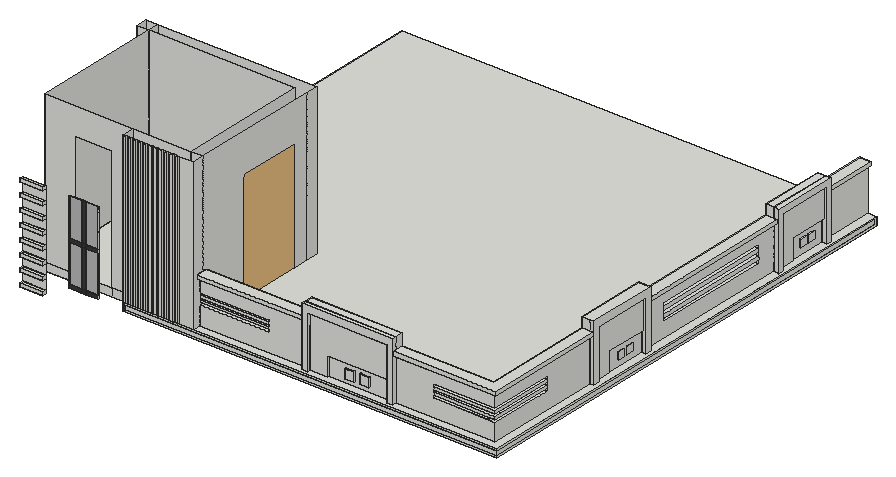
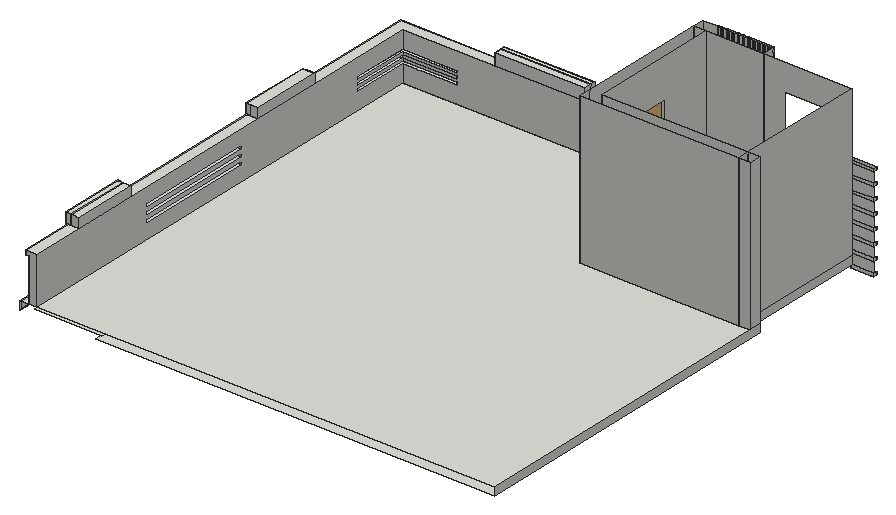
# SketchUp Ruby script. Lengths in inches.
U = 1.inch
M = Sketchup.active_model
def pt(a) = Geom::Point3d.new(a.map { |v| v * U })
def face(e, loops, mat)
  f = e.add_face(loops[0].map { |a| pt(a) })
  loops[1..].each { |l| e.add_face(l.map { |a| pt(a) }).erase! }
  f.material = f.back_material = mat if mat
  f
end
# faces: each face lists its corners as indices into pts; further lists are holes
def faces(e, pts, list, mat = nil) = list.each { |f| face(e, (f[0].is_a?(Array) ? f : [f]).map { |l| l.map { |i| pts[i] } }, mat) }
# xy, xz, yz: faces in a plane at the given z, y or x. An outline is a flat list of corners, or four numbers for a rectangle; further outlines are holes
def ring(l) = l.size == 4 ? [[l[0], l[1]], [l[2], l[1]], [l[2], l[3]], [l[0], l[3]]] : l.each_slice(2).to_a
def flat(e, list, mat, &to3) = list.each { |f| face(e, (f[0].is_a?(Array) ? f : [f]).map { |l| ring(l).map { |u, v| to3.(u, v) } }, mat) }
def xy(e, z, list, mat = nil) = flat(e, list, mat) { |x, y| [x, y, z] }
def xz(e, y, list, mat = nil) = flat(e, list, mat) { |x, z| [x, y, z] }
def yz(e, x, list, mat = nil) = flat(e, list, mat) { |y, z| [x, y, z] }
def lines(e, pts, list) = list.each { |a, b| e.add_line(pt(pts[a]), pt(pts[b])) }
# prism: a flat outline (further loops are holes) pulled along v
def prism(e, loops, v, mat = nil)
  f = face(e, loops, mat); d = Geom::Vector3d.new(v.map { |x| x * U })
  f.pushpull(f.normal.samedirection?(d) ? d.length : -d.length)
end
def box(e, o, s, mat = nil) = prism(e, [[o, [o[0] + s[0], o[1], o[2]], [o[0] + s[0], o[1] + s[1], o[2]], [o[0], o[1] + s[1], o[2]]]], [0, 0, s[2]], mat)
def at(x, y, z, deg = 0) = Geom::Transformation.translation(pt([x, y, z])) * Geom::Transformation.rotation(ORIGIN, Z_AXIS, deg.degrees)
def axes(o, x, y, z) = Geom::Transformation.new([*x, 0, *y, 0, *z, 0, *pt(o).to_a, 1])
def part(name) = M.definitions.add(name)
# library, detail: a bought-in or finely detailed component or shape, given as its bounding box
def library(name, o, s) = part(name).tap { |d| box(d.entities, o, s) }
def detail(e, o, s) = box(e.add_group.entities, o, s)
def put(e, d, t, mat = nil) = e.add_instance(d, t).tap { |i| i.material = mat if mat }
def group(e, t, mat = nil) = e.add_group.tap { |g| g.transformation = t; g.material = mat if mat }.entities
root = M.entities
M.materials.add("[Color M07]").color = [58, 58, 58]
M.materials.add("[Mirror 01]").color = [185, 185, 185]
c1 = library("Door 243 053",[-21.6,-2.79,-0.07],[43.2,5.58,82.64])
xy(root,237.07,[[7.9375,22.5,25.22,25.1875]])
xy(root,239.42,[[7.9375,22.5,25.22,25.1875]])
xy(root,244.8125,[[357.6875,206.85,364.9375,220.375],[364.9375,206.85,367,220.375]])
xy(root,246,[[84.23,24.75,84.23,25.1875,367.9375,25.1875,367.9375,385.1875,368.375,385.1875,368.375,24.75],[84.23,25.1875,137.39,34.1875],[196.07,25.625,215.37,31.1875],[327.58,25.625,343.4,25.625,343.4,28.1875,359.0625,28.1875,359.0625,31.1875,327.58,31.1875],[359.0625,28.1875,361.9375,31.1875],
  [361.9375,28.1875,364.9375,31.1875],[137.39,31.1875,137.39,34.1875,84.23,34.1875,84.23,133.1875,310.9375,133.1875,310.9375,379.1875,361.9375,379.1875,361.9375,34.1875,343.4,34.1875,343.4,36.25,327.58,36.25,327.58,31.1875,215.37,31.1875,215.37,36.25,196.07,36.25,196.07,31.1875],[196.07,31.1875,215.37,36.25],[327.58,31.1875,361.9375,31.1875,361.9375,34.1875,343.4,34.1875,343.4,36.25,327.58,36.25],[16.9375,34.1875,84.23,133.1875],
  [[7.9375,133.1875,310.9375,385.1875],[16.9375,142.1875,301.9375,376.1875]]])
xy(root,247,[[85.23,24.75,368.375,24.75,368.375,384.1875,367.9375,384.1875,367.9375,25.1875,85.23,25.1875],[364.9375,70.91,367,84.5]])
xy(root,247.11,[[52.28,25.1875,55.28,26.1875],[43.02,25.6875,52.28,26.1875],[55.28,25.6875,64.8,26.1875]])
xy(root,247.11,[[43.02,25.1875,52.28,25.6875],[55.28,25.1875,64.8,25.6875]],"[Color M07]")
xy(root,247.25,[[7.9375,22.5,25.22,25.1875]])
xy(root,249.6,[[7.9375,22.5,25.22,25.1875]])
xy(root,249.74,[[52.28,25.1875,55.28,26.1875],[43.02,25.6875,52.28,26.1875],[55.28,25.6875,64.8,26.1875]])
xy(root,249.74,[[43.02,25.1875,52.28,25.6875],[55.28,25.1875,64.8,25.6875]],"[Color M07]")
xy(root,251,[[84.23,24.75,85.23,25.1875],[85.23,24.75,85.23,25.1875,367.9375,25.1875,367.9375,384.1875,368.375,384.1875,368.375,24.75]])
xy(root,252,[[84.23,24.75,85.23,25.1875],[85.23,24.75,368.375,24.75,368.375,385.1875,367.9375,385.1875,367.9375,25.1875,85.23,25.1875],[84.23,25.1875,128.39,34.1875],[128.39,25.1875,137.39,34.1875],[137.39,25.1875,367.9375,25.1875,367.9375,385.1875,361.9375,385.1875,361.9375,344.85,366.25,344.85,366.25,341.21,361.9375,341.21,361.9375,312.14,363.5,312.14,363.5,299.05,366.25,299.05,366.25,295.41,361.9375,295.41,361.9375,174.68,365.1875,174.68,365.1875,170.17,361.9375,170.17,361.9375,137.91,363.125,137.91,363.125,125.76,365.1875,125.76,365.1875,121.25,361.9375,121.25,361.9375,31.1875,286.38,31.1875,286.38,27.9375,282.22,27.9375,282.22,31.1875,235.34,31.1875,235.34,30.125,221.92,30.125,221.92,27.9375,217.77,27.9375,217.77,31.1875,137.39,31.1875],
  [217.77,27.9375,221.92,31.1875],[282.22,27.9375,286.38,31.1875],[221.92,30.125,221.92,31.1875,137.39,31.1875,137.39,37.1875,361.9375,37.1875,361.9375,31.1875,235.34,31.1875,235.34,30.125],[16.9375,34.1875,84.23,133.1875],[84.23,34.1875,128.39,133.1875],
  [128.39,34.1875,137.39,73.1875],[137.39,37.1875,355.9375,37.1875,355.9375,385.1875,7.9375,385.1875,7.9375,142.1875,137.39,142.1875,137.39,121.1875,128.39,121.1875,128.39,73.1875,137.39,73.1875],[355.9375,37.1875,355.9375,385.1875,361.9375,385.1875,361.9375,312.14,363.5,312.14,363.5,299.05,361.9375,299.05,361.9375,137.91,363.125,137.91,363.125,125.76,361.9375,125.76,361.9375,37.1875],[128.39,121.1875,137.39,133.1875],[361.9375,121.25,365.1875,125.76],
  [7.9375,133.1875,16.9375,142.1875],[16.9375,133.1875,137.39,142.1875],[361.9375,170.17,365.1875,174.68],[361.9375,295.41,366.25,299.05],[361.9375,341.21,366.25,344.85]])
xy(root,252.6875,[[84.23,24.25,86.79,25.1875],[88.1,24.25,90.66,25.1875],[91.98,24.25,94.54,25.1875],[95.85,24.25,98.41,25.1875],[99.73,24.25,102.29,25.1875],
  [103.6,24.25,106.16,25.1875],[107.48,24.25,110.04,25.1875],[111.35,24.25,113.91,25.1875],[115.54,24.25,118.1,25.1875],[119.73,24.25,122.29,25.1875],
  [123.91,24.25,126.48,25.1875]])
xy(root,255.53,[[248.55,30.125,255.49,31.1875],[259.49,30.125,266.43,31.1875]])
xy(root,257.23,[[361.9375,146.76,363.125,152.14],[361.9375,154.89,363.125,160.26]])
xy(root,257.44,[[7.9375,22.5,25.22,25.1875]])
xy(root,257.85,[[361.9375,319.64,363.5,325.27],[361.9375,327.39,363.5,333.02]])
xy(root,259.79,[[7.9375,22.5,25.22,25.1875]])
xy(root,262.46,[[248.55,30.125,255.49,31.1875],[259.49,30.125,266.43,31.1875]])
xy(root,262.6,[[361.9375,146.76,363.125,152.14],[361.9375,154.89,363.125,160.26]])
xy(root,263.41,[[355.9375,190.16,361.9375,281.48]])
xy(root,263.48,[[361.9375,319.64,363.5,325.27],[361.9375,327.39,363.5,333.02]])
xy(root,265.05,[[314.9375,31.1875,355.9375,37.1875],[355.9375,31.1875,361.9375,80.6875]])
xy(root,266.06,[[355.9375,190.16,361.9375,281.48]])
xy(root,266.25,[[235.34,30.125,282.22,31.1875]])
xy(root,266.44,[[137.39,31.1875,189.76,34.1875]])
xy(root,267.01,[[314.9375,31.1875,355.9375,37.1875],[355.9375,31.1875,361.9375,80.6875]])
xy(root,267.0625,[[361.9375,137.91,363.125,170.17]])
xy(root,267.63,[[7.9375,22.5,25.22,25.1875]])
xy(root,267.875,[[361.9375,312.14,363.5,341.21]])
xy(root,268.03,[[137.39,31.1875,189.76,34.1875]])
xy(root,268.71,[[355.9375,190.16,361.9375,281.48]])
xy(root,268.97,[[314.9375,31.1875,361.9375,37.1875],[355.9375,37.1875,361.9375,80.6875]])
xy(root,269.62,[[137.39,31.1875,189.76,34.1875]])
xy(root,269.98,[[7.9375,22.5,25.22,25.1875]])
xy(root,270.94,[[314.9375,31.1875,361.9375,37.1875],[355.9375,37.1875,361.9375,80.6875]])
xy(root,271.2,[[137.39,31.1875,189.76,34.1875]])
xy(root,271.36,[[355.9375,190.16,361.9375,281.48]])
xy(root,272.79,[[137.39,31.1875,189.76,34.1875]])
xy(root,272.9,[[314.9375,31.1875,355.9375,37.1875],[355.9375,31.1875,361.9375,80.6875]])
xy(root,274.01,[[355.9375,190.16,361.9375,281.48]])
xy(root,274.38,[[137.39,31.1875,189.76,34.1875]])
xy(root,274.86,[[314.9375,31.1875,355.9375,37.1875],[355.9375,31.1875,361.9375,80.6875]])
xy(root,276.66,[[355.9375,190.16,361.9375,281.48]])
xy(root,277.82,[[7.9375,22.5,25.22,25.1875]])
xy(root,278.42,[[52.28,25.1875,55.28,26.1875],[43.02,25.6875,52.28,26.1875],[55.28,25.6875,64.8,26.1875]])
xy(root,278.42,[[43.02,25.1875,52.28,25.6875],[55.28,25.1875,64.8,25.6875]],"[Color M07]")
xy(root,280.17,[[7.9375,22.5,25.22,25.1875]])
xy(root,281.05,[[52.28,25.1875,55.28,26.1875],[43.02,25.5,52.28,25.6875],[55.28,25.5,64.8,25.6875],[43.02,25.6875,52.28,26.1875],[55.28,25.6875,64.8,26.1875]])
xy(root,281.05,[[43.02,25.1875,52.28,25.5],[55.28,25.1875,64.8,25.5]],"[Color M07]")
xy(root,285,[[137.39,28.6875,217.77,31.1875],[286.38,28.6875,364.4375,31.1875],[361.9375,31.1875,364.4375,121.25],[361.9375,174.68,364.4375,295.41],[361.9375,344.85,364.4375,385.1875]])
xy(root,288,[[7.9375,22.5,25.22,25.1875],[137.39,28.6875,217.77,37.1875],[286.38,28.6875,364.4375,28.6875,364.4375,121.25,355.9375,121.25,355.9375,37.1875,286.38,37.1875],[217.77,31.1875,286.38,37.1875],[355.9375,121.25,361.9375,174.68],
  [355.9375,174.68,364.4375,295.41],[355.9375,344.85,364.4375,385.1875]])
xy(root,289.87,[[363.125,125.76,365.1875,170.17]])
xy(root,290.35,[[7.9375,22.5,25.22,25.1875]])
xy(root,290.6875,[[361.9375,299.05,363.5,341.21],[363.5,299.05,366.25,341.21]])
xy(root,291.53,[[221.92,27.9375,282.22,30.125]])
xy(root,295.4375,[[355.9375,121.25,365.1875,174.68],[355.9375,295.41,361.9375,344.85],[361.9375,295.41,366.25,344.85]])
xy(root,296.9375,[[217.77,27.9375,286.38,31.1875],[217.77,31.1875,286.38,37.1875]])
xy(root,298.19,[[7.9375,22.5,25.22,25.1875]])
xy(root,300.54,[[7.9375,22.5,25.22,25.1875]])
xy(root,308.38,[[7.9375,22.5,25.22,25.1875]])
xz(root,22.5,[[7.9375,237.07,25.22,239.42],[7.9375,247.25,25.22,249.6],[7.9375,257.44,25.22,259.79],[7.9375,267.63,25.22,269.98],[7.9375,277.82,25.22,280.17],
  [7.9375,288,25.22,290.35],[7.9375,298.19,25.22,300.54],[7.9375,308.38,25.22,310.73]])
xz(root,24.25,[[84.23,252.6875,86.79,366],[88.1,252.6875,90.66,366],[91.98,252.6875,94.54,366],[95.85,252.6875,98.41,366],[99.73,252.6875,102.29,366],
  [103.6,252.6875,106.16,366],[107.48,252.6875,110.04,366],[111.35,252.6875,113.91,366],[115.54,252.6875,118.1,366],[119.73,252.6875,122.29,366],
  [123.91,252.6875,126.48,366]])
xz(root,24.75,[[84.23,246,368.375,246,368.375,247,85.23,247,85.23,251,84.23,251],[84.23,251,85.23,252],[85.23,251,368.375,252]])
xz(root,25.1875,[[7.9375,237.07,25.22,239.42],[7.9375,239.42,25.22,247.25],[85.23,247,367.9375,251],[7.9375,247.25,25.22,249.6],[7.9375,249.6,25.22,257.44],
  [84.23,251,85.23,252],[84.23,252,137.39,252,137.39,366,126.48,366,126.48,252.6875,123.91,252.6875,123.91,366,122.29,366,122.29,252.6875,119.73,252.6875,119.73,366,118.1,366,118.1,252.6875,115.54,252.6875,115.54,366,113.91,366,113.91,252.6875,111.35,252.6875,111.35,366,110.04,366,110.04,252.6875,107.48,252.6875,107.48,366,106.16,366,106.16,252.6875,103.6,252.6875,103.6,366,102.29,366,102.29,252.6875,99.73,252.6875,99.73,366,98.41,366,98.41,252.6875,95.85,252.6875,95.85,366,94.54,366,94.54,252.6875,91.98,252.6875,91.98,366,90.66,366,90.66,252.6875,88.1,252.6875,88.1,366,86.79,366,86.79,252.6875,84.23,252.6875],[84.23,252.6875,86.79,366],[88.1,252.6875,90.66,366],[91.98,252.6875,94.54,366],
  [95.85,252.6875,98.41,366],[99.73,252.6875,102.29,366],[103.6,252.6875,106.16,366],[107.48,252.6875,110.04,366],[111.35,252.6875,113.91,366],
  [115.54,252.6875,118.1,366],[119.73,252.6875,122.29,366],[123.91,252.6875,126.48,366],[7.9375,257.44,25.22,259.79],[7.9375,259.79,25.22,267.63],
  [7.9375,267.63,25.22,269.98],[7.9375,269.98,25.22,277.82],[7.9375,277.82,25.22,280.17],[7.9375,280.17,25.22,288],[7.9375,288,25.22,290.35],
  [7.9375,290.35,25.22,298.19],[7.9375,298.19,25.22,300.54],[7.9375,300.54,25.22,308.38],[7.9375,308.38,25.22,310.73]])
xz(root,25.1875,[[43.02,247.11,52.28,249.74],[52.28,247.11,55.28,249.74],[55.28,247.11,64.8,249.74],[52.28,249.74,55.28,278.42],[43.02,278.42,52.28,281.05],
  [52.28,278.42,55.28,281.05],[55.28,278.42,64.8,281.05],[52.28,281.05,55.28,309.73]],"[Color M07]")
xz(root,25.5,[[43.02,281.05,52.28,309.73],[55.28,281.05,64.8,309.73]],"[Mirror 01]")
xz(root,25.6875,[[43.02,281.05,52.28,309.73],[55.28,281.05,64.8,309.73]])
xz(root,25.6875,[[43.02,249.74,52.28,278.42],[55.28,249.74,64.8,278.42]],"[Mirror 01]")
xz(root,26.1875,[[43.02,247.11,52.28,249.74],[52.28,247.11,55.28,249.74],[55.28,247.11,64.8,249.74],[52.28,249.74,55.28,278.42],[43.02,278.42,52.28,281.05],
  [52.28,278.42,55.28,281.05],[55.28,278.42,64.8,281.05],[52.28,281.05,55.28,309.73]],"[Color M07]")
xz(root,26.1875,[[43.02,249.74,52.28,278.42],[55.28,249.74,64.8,278.42],[43.02,281.05,52.28,309.73],[55.28,281.05,64.8,309.73]],"[Mirror 01]")
xz(root,27.9375,[[217.77,252,221.92,252,221.92,291.53,282.22,291.53,282.22,252,286.38,252,286.38,296.9375,217.77,296.9375]])
xz(root,28.6875,[[137.39,285,217.77,288],[286.38,285,364.4375,288]])
xz(root,30.125,[[221.92,252,235.34,252,235.34,266.25,282.22,266.25,282.22,291.53,221.92,291.53],[248.55,255.53,255.49,262.46],[259.49,255.53,266.43,262.46]])
xz(root,31.1875,[[137.39,252,217.77,252,217.77,285,137.39,285,137.39,274.38,189.76,274.38,189.76,266.44,137.39,266.44],[217.77,252,217.77,288,286.38,288,286.38,252,282.22,252,282.22,283.84,221.92,283.84,221.92,252],[[235.34,252,282.22,266.25],[248.55,255.53,255.49,262.46],[259.49,255.53,266.43,262.46]],[286.38,252,361.9375,252,361.9375,265.05,314.9375,265.05,314.9375,274.86,361.9375,274.86,361.9375,285,286.38,285],[314.9375,267.01,361.9375,268.97],
  [137.39,268.03,189.76,269.62],[314.9375,270.94,361.9375,272.9],[137.39,271.2,189.76,272.79],[217.77,288,286.38,296.9375]])
xz(root,34.1875,[[16.9375,246,39.8125,252],[39.8125,246,68,252],[68,246,84.23,252],[16.9375,252,16.9375,366,84.23,366,84.23,252,68,252,68,345.39,39.8125,345.39,39.8125,252],[84.23,252,128.39,366],
  [128.39,252,137.39,366],[137.39,266.44,189.76,268.03],[137.39,269.62,189.76,271.2],[137.39,272.79,189.76,274.38]])
xz(root,37.1875,[[137.39,252,137.39,288,355.9375,288,355.9375,274.86,314.9375,274.86,314.9375,272.9,355.9375,272.9,355.9375,270.94,314.9375,270.94,314.9375,268.97,355.9375,268.97,355.9375,267.01,314.9375,267.01,314.9375,265.05,355.9375,265.05,355.9375,252],[314.9375,268.97,355.9375,270.94],[217.77,288,286.38,296.9375]])
xz(root,73.1875,[[128.39,252,137.39,336]])
xz(root,80.6875,[[355.9375,265.05,361.9375,267.01],[355.9375,268.97,361.9375,270.94],[355.9375,272.9,361.9375,274.86]])
xz(root,121.1875,[[128.39,252,137.39,336]])
xz(root,121.25,[[361.9375,252,365.1875,252,365.1875,288,364.4375,288,364.4375,285,361.9375,285],[361.9375,285,364.4375,288],[355.9375,288,361.9375,295.4375],[361.9375,288,365.1875,295.4375]])
xz(root,125.76,[[361.9375,252,363.125,283.49],[363.125,252,365.1875,289.87]])
xz(root,133.1875,[[7.9375,246,16.9375,252],[16.9375,246,84.23,252],[7.9375,252,16.9375,366],[16.9375,252,128.39,366]])
xz(root,137.91,[[361.9375,252,363.125,267.0625]])
xz(root,142.1875,[[7.9375,252,16.9375,366],[16.9375,252,137.39,366]])
xz(root,146.76,[[361.9375,257.23,363.125,262.6]])
xz(root,152.14,[[361.9375,257.23,363.125,262.6]])
xz(root,154.89,[[361.9375,257.23,363.125,262.6]])
xz(root,160.26,[[361.9375,257.23,363.125,262.6]])
xz(root,170.17,[[361.9375,252,365.1875,252,365.1875,289.87,363.125,289.87,363.125,267.0625,361.9375,267.0625],[361.9375,267.0625,363.125,283.49]])
xz(root,174.68,[[361.9375,252,361.9375,285,364.4375,285,364.4375,288,365.1875,288,365.1875,252],[361.9375,285,364.4375,288],[355.9375,288,361.9375,295.4375],[361.9375,288,365.1875,295.4375]])
xz(root,190.16,[[355.9375,263.41,361.9375,266.06],[355.9375,268.71,361.9375,271.36],[355.9375,274.01,361.9375,276.66]])
xz(root,281.48,[[355.9375,263.41,361.9375,266.06],[355.9375,268.71,361.9375,271.36],[355.9375,274.01,361.9375,276.66]])
xz(root,295.41,[[361.9375,252,366.25,252,366.25,288,364.4375,288,364.4375,285,361.9375,285],[361.9375,285,364.4375,288],[355.9375,288,361.9375,295.4375],[361.9375,288,366.25,295.4375]])
xz(root,299.05,[[361.9375,252,363.5,288],[363.5,252,366.25,290.6875],[361.9375,288,363.5,290.6875]])
xz(root,312.14,[[361.9375,252,363.5,267.875]])
xz(root,319.64,[[361.9375,257.85,363.5,263.48]])
xz(root,325.27,[[361.9375,257.85,363.5,263.48]])
xz(root,327.39,[[361.9375,257.85,363.5,263.48]])
xz(root,333.02,[[361.9375,257.85,363.5,263.48]])
xz(root,341.21,[[361.9375,252,366.25,252,366.25,290.6875,363.5,290.6875,363.5,267.875,361.9375,267.875],[361.9375,267.875,363.5,288],[361.9375,288,363.5,290.6875]])
xz(root,344.85,[[361.9375,252,361.9375,285,364.4375,285,364.4375,288,366.25,288,366.25,252],[361.9375,285,364.4375,288],[355.9375,288,361.9375,295.4375],[361.9375,288,366.25,295.4375]])
xz(root,384.1875,[[367.9375,247,368.375,251]])
xz(root,385.1875,[[367.9375,246,368.375,252],[355.9375,252,355.9375,288,364.4375,288,364.4375,285,361.9375,285,361.9375,252]])
yz(root,7.9375,[[22.5,237.07,25.1875,239.42],[133.1875,246,385.1875,252],[22.5,247.25,25.1875,249.6],[133.1875,252,142.1875,366],[22.5,257.44,25.1875,259.79],
  [22.5,267.63,25.1875,269.98],[22.5,277.82,25.1875,280.17],[22.5,288,25.1875,290.35],[22.5,298.19,25.1875,300.54],[22.5,308.38,25.1875,310.73]])
yz(root,16.9375,[[34.1875,246,133.1875,252],[34.1875,252,133.1875,366],[133.1875,252,142.1875,366]])
yz(root,25.22,[[22.5,237.07,25.1875,239.42],[22.5,247.25,25.1875,249.6],[22.5,257.44,25.1875,259.79],[22.5,267.63,25.1875,269.98],[22.5,277.82,25.1875,280.17],
  [22.5,288,25.1875,290.35],[22.5,298.19,25.1875,300.54],[22.5,308.38,25.1875,310.73]])
yz(root,43.02,[[25.1875,247.11,26.1875,249.74],[25.6875,249.74,26.1875,278.42],[25.1875,278.42,26.1875,281.05],[25.5,281.05,25.6875,309.73],[25.6875,281.05,26.1875,309.73]])
yz(root,43.02,[[25.1875,249.74,25.6875,278.42],[25.1875,281.05,25.5,309.73]],"[Color M07]")
yz(root,52.28,[[25.1875,247.11,26.1875,249.74],[25.6875,249.74,26.1875,278.42],[25.1875,278.42,26.1875,281.05],[25.5,281.05,25.6875,309.73],[25.6875,281.05,26.1875,309.73]])
yz(root,52.28,[[25.1875,249.74,25.6875,278.42],[25.1875,281.05,25.5,309.73]],"[Color M07]")
yz(root,55.28,[[25.1875,247.11,26.1875,249.74],[25.6875,249.74,26.1875,278.42],[25.1875,278.42,26.1875,281.05],[25.5,281.05,25.6875,309.73],[25.6875,281.05,26.1875,309.73]])
yz(root,55.28,[[25.1875,249.74,25.6875,278.42],[25.1875,281.05,25.5,309.73]],"[Color M07]")
yz(root,64.8,[[25.1875,247.11,26.1875,249.74],[25.6875,249.74,26.1875,278.42],[25.1875,278.42,26.1875,281.05],[25.5,281.05,25.6875,309.73],[25.6875,281.05,26.1875,309.73]])
yz(root,64.8,[[25.1875,249.74,25.6875,278.42],[25.1875,281.05,25.5,309.73]],"[Color M07]")
yz(root,84.23,[[24.75,246,25.1875,251],[25.1875,246,34.1875,252],[34.1875,246,133.1875,252],[24.75,251,25.1875,252],[25.1875,252,34.1875,366],
  [24.25,252.6875,25.1875,366]])
yz(root,85.23,[[24.75,247,25.1875,251]])
yz(root,86.79,[[24.25,252.6875,25.1875,366]])
yz(root,88.1,[[24.25,252.6875,25.1875,366]])
yz(root,90.66,[[24.25,252.6875,25.1875,366]])
yz(root,91.98,[[24.25,252.6875,25.1875,366]])
yz(root,94.54,[[24.25,252.6875,25.1875,366]])
yz(root,95.85,[[24.25,252.6875,25.1875,366]])
yz(root,98.41,[[24.25,252.6875,25.1875,366]])
yz(root,99.73,[[24.25,252.6875,25.1875,366]])
yz(root,102.29,[[24.25,252.6875,25.1875,366]])
yz(root,103.6,[[24.25,252.6875,25.1875,366]])
yz(root,106.16,[[24.25,252.6875,25.1875,366]])
yz(root,107.48,[[24.25,252.6875,25.1875,366]])
yz(root,110.04,[[24.25,252.6875,25.1875,366]])
yz(root,111.35,[[24.25,252.6875,25.1875,366]])
yz(root,113.91,[[24.25,252.6875,25.1875,366]])
yz(root,115.54,[[24.25,252.6875,25.1875,366]])
yz(root,118.1,[[24.25,252.6875,25.1875,366]])
yz(root,119.73,[[24.25,252.6875,25.1875,366]])
yz(root,122.29,[[24.25,252.6875,25.1875,366]])
yz(root,123.91,[[24.25,252.6875,25.1875,366]])
yz(root,126.48,[[24.25,252.6875,25.1875,366]])
yz(root,128.39,[[34.1875,252,34.1875,366,133.1875,366,133.1875,252,121.1875,252,121.1875,336,73.1875,336,73.1875,252]])
yz(root,137.39,[[25.1875,252,31.1875,252,31.1875,266.44,34.1875,266.44,34.1875,268.03,31.1875,268.03,31.1875,269.62,34.1875,269.62,34.1875,271.2,31.1875,271.2,31.1875,272.79,34.1875,272.79,34.1875,274.38,31.1875,274.38,31.1875,285,28.6875,285,28.6875,288,34.1875,288,34.1875,366,25.1875,366],[31.1875,252,34.1875,266.44],[34.1875,252,37.1875,288],[37.1875,252,73.1875,252,73.1875,336,121.1875,336,121.1875,252,133.1875,252,133.1875,366,34.1875,366,34.1875,288,37.1875,288],[133.1875,252,142.1875,366],
  [31.1875,268.03,34.1875,269.62],[31.1875,271.2,34.1875,272.79],[31.1875,274.38,34.1875,274.38,34.1875,288,28.6875,288,28.6875,285,31.1875,285]])
yz(root,189.76,[[31.1875,266.44,34.1875,268.03],[31.1875,269.62,34.1875,271.2],[31.1875,272.79,34.1875,274.38]])
yz(root,217.77,[[27.9375,252,27.9375,288,28.6875,288,28.6875,285,31.1875,285,31.1875,252],[28.6875,285,31.1875,288],[27.9375,288,31.1875,296.9375],[31.1875,288,37.1875,296.9375]])
yz(root,221.92,[[27.9375,252,30.125,291.53],[30.125,252,31.1875,283.84]])
yz(root,235.34,[[30.125,252,31.1875,266.25]])
yz(root,248.55,[[30.125,255.53,31.1875,262.46]])
yz(root,255.49,[[30.125,255.53,31.1875,262.46]])
yz(root,259.49,[[30.125,255.53,31.1875,262.46]])
yz(root,266.43,[[30.125,255.53,31.1875,262.46]])
yz(root,282.22,[[27.9375,252,27.9375,291.53,30.125,291.53,30.125,266.25,31.1875,266.25,31.1875,252],[30.125,266.25,31.1875,283.84]])
yz(root,286.38,[[27.9375,252,31.1875,252,31.1875,285,28.6875,285,28.6875,288,27.9375,288],[28.6875,285,31.1875,288],[27.9375,288,31.1875,296.9375],[31.1875,288,37.1875,296.9375]])
yz(root,314.9375,[[31.1875,265.05,37.1875,267.01],[31.1875,268.97,37.1875,270.94],[31.1875,272.9,37.1875,274.86]])
yz(root,355.9375,[[[37.1875,252,37.1875,265.05,80.6875,265.05,80.6875,267.01,37.1875,267.01,37.1875,268.97,80.6875,268.97,80.6875,270.94,37.1875,270.94,37.1875,272.9,80.6875,272.9,80.6875,274.86,37.1875,274.86,37.1875,288,385.1875,288,385.1875,252],[190.16,274.01,281.48,276.66],[190.16,268.71,281.48,271.36],[190.16,263.41,281.48,266.06]],[121.25,288,174.68,295.4375],[295.41,288,344.85,295.4375]])
yz(root,361.9375,[[31.1875,252,121.25,252,121.25,285,31.1875,285,31.1875,274.86,80.6875,274.86,80.6875,265.05,31.1875,265.05],[121.25,252,121.25,288,174.68,288,174.68,252,170.17,252,170.17,283.49,125.76,283.49,125.76,252],[[137.91,252,170.17,267.0625],[146.76,257.23,152.14,262.6],[154.89,257.23,160.26,262.6]],[[174.68,252,295.41,285],[190.16,263.41,281.48,276.66]],[295.41,252,299.05,288],
  [[312.14,252,341.21,267.875],[319.64,257.85,325.27,263.48],[327.39,257.85,333.02,263.48]],[341.21,252,344.85,288],[344.85,252,385.1875,285],[190.16,266.06,281.48,268.71],[31.1875,267.01,80.6875,268.97],
  [31.1875,270.94,80.6875,272.9],[190.16,271.36,281.48,274.01],[295.41,288,299.05,288,299.05,290.6875,341.21,290.6875,341.21,288,344.85,288,344.85,295.4375,295.41,295.4375]])
yz(root,363.125,[[125.76,252,137.91,252,137.91,267.0625,170.17,267.0625,170.17,289.87,125.76,289.87],[146.76,257.23,152.14,262.6],[154.89,257.23,160.26,262.6]])
yz(root,363.5,[[299.05,252,312.14,252,312.14,267.875,341.21,267.875,341.21,290.6875,299.05,290.6875],[319.64,257.85,325.27,263.48],[327.39,257.85,333.02,263.48]])
yz(root,364.4375,[[28.6875,285,121.25,288],[174.68,285,295.41,288],[344.85,285,385.1875,288]])
yz(root,365.1875,[[121.25,252,125.76,252,125.76,289.87,170.17,289.87,170.17,252,174.68,252,174.68,295.4375,121.25,295.4375]])
yz(root,366.25,[[295.41,252,299.05,252,299.05,290.6875,341.21,290.6875,341.21,252,344.85,252,344.85,295.4375,295.41,295.4375]])
yz(root,367.9375,[[25.1875,247,384.1875,251]])
yz(root,368.375,[[24.75,246,385.1875,246,385.1875,252,24.75,252,24.75,251,384.1875,251,384.1875,247,24.75,247]])
p = [[355.9375,37.1875,272.9],[355.9375,37.1875,274.86],[355.9375,37.1875,265.05],[355.9375,37.1875,267.01]]
lines(root,p,[[0,1],[2,3]])
put(root,c1,axes([134.32,96.99,252.07],[0,1.10192,0],[-1.10192,0,0],[0,0,1.01657]))
